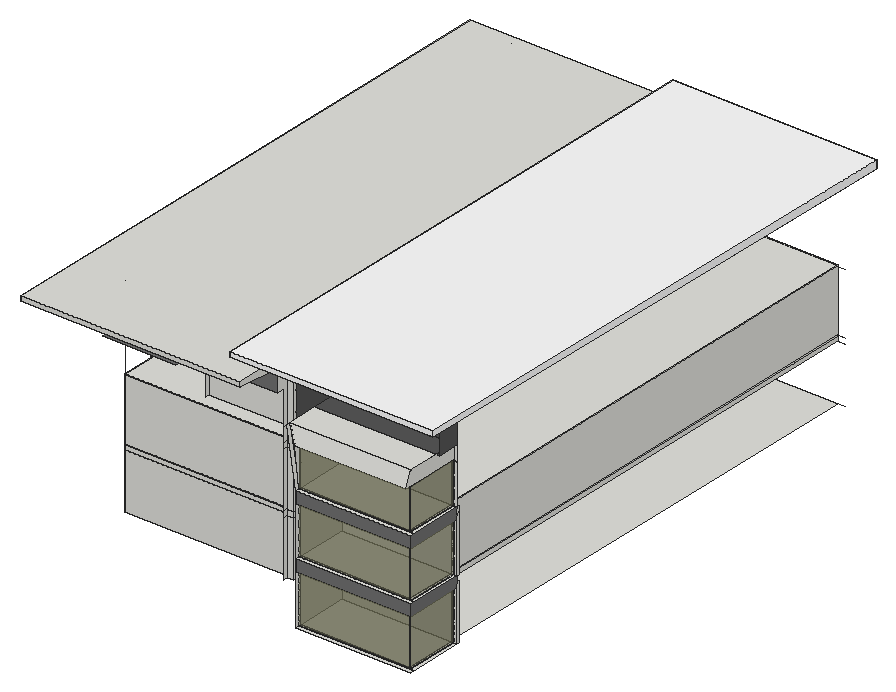
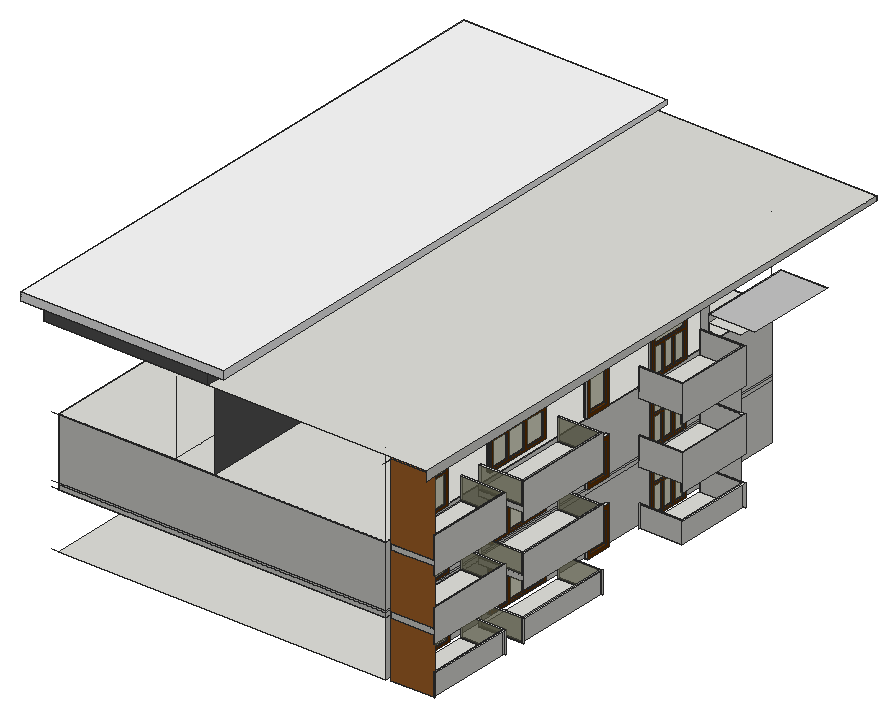
# SketchUp Ruby script. Lengths in inches.
U = 1.inch
M = Sketchup.active_model
def pt(a) = Geom::Point3d.new(a.map { |v| v * U })
def face(e, loops, mat)
  f = e.add_face(loops[0].map { |a| pt(a) })
  loops[1..].each { |l| e.add_face(l.map { |a| pt(a) }).erase! }
  f.material = f.back_material = mat if mat
  f
end
# faces: each face lists its corners as indices into pts; further lists are holes
def faces(e, pts, list, mat = nil) = list.each { |f| face(e, (f[0].is_a?(Array) ? f : [f]).map { |l| l.map { |i| pts[i] } }, mat) }
# xy, xz, yz: faces in a plane at the given z, y or x. An outline is a flat list of corners, or four numbers for a rectangle; further outlines are holes
def ring(l) = l.size == 4 ? [[l[0], l[1]], [l[2], l[1]], [l[2], l[3]], [l[0], l[3]]] : l.each_slice(2).to_a
def flat(e, list, mat, &to3) = list.each { |f| face(e, (f[0].is_a?(Array) ? f : [f]).map { |l| ring(l).map { |u, v| to3.(u, v) } }, mat) }
def xy(e, z, list, mat = nil) = flat(e, list, mat) { |x, y| [x, y, z] }
def xz(e, y, list, mat = nil) = flat(e, list, mat) { |x, z| [x, y, z] }
def yz(e, x, list, mat = nil) = flat(e, list, mat) { |y, z| [x, y, z] }
def lines(e, pts, list) = list.each { |a, b| e.add_line(pt(pts[a]), pt(pts[b])) }
# prism: a flat outline (further loops are holes) pulled along v
def prism(e, loops, v, mat = nil)
  f = face(e, loops, mat); d = Geom::Vector3d.new(v.map { |x| x * U })
  f.pushpull(f.normal.samedirection?(d) ? d.length : -d.length)
end
def box(e, o, s, mat = nil) = prism(e, [[o, [o[0] + s[0], o[1], o[2]], [o[0] + s[0], o[1] + s[1], o[2]], [o[0], o[1] + s[1], o[2]]]], [0, 0, s[2]], mat)
def at(x, y, z, deg = 0) = Geom::Transformation.translation(pt([x, y, z])) * Geom::Transformation.rotation(ORIGIN, Z_AXIS, deg.degrees)
def axes(o, x, y, z) = Geom::Transformation.new([*x, 0, *y, 0, *z, 0, *pt(o).to_a, 1])
def part(name) = M.definitions.add(name)
# library, detail: a bought-in or finely detailed component or shape, given as its bounding box
def library(name, o, s) = part(name).tap { |d| box(d.entities, o, s) }
def detail(e, o, s) = box(e.add_group.entities, o, s)
def put(e, d, t, mat = nil) = e.add_instance(d, t).tap { |i| i.material = mat if mat }
def group(e, t, mat = nil) = e.add_group.tap { |g| g.transformation = t; g.material = mat if mat }.entities
root = M.entities
M.materials.add("[Color A08]").color = [102, 50, 0]
M.materials.add("[Color M00]").color = [255, 255, 255]
M.materials.add("[Color M02]").color = [198, 198, 198]
M.materials.add("[Color M05]").color = [114, 114, 114]
M.materials.add("[Color M06]").color = [86, 86, 86]
M.materials.add("[Translucent Glass Gray]").color = [128, 128, 99]
M.materials["[Translucent Glass Gray]"].alpha = 0.5
M.materials.add("[Translucent Glass Gray]1").color = [128, 128, 95]
M.materials["[Translucent Glass Gray]1"].alpha = 0.5
M.materials.add("[Wood Bamboo]").color = [177, 105, 43]
c1 = part("Group\#2")
xy(c1.entities,0,[[0,0,3.1875,51.25]],"[Color A08]")
xy(c1.entities,5.52,[[0,5.52,3.1875,45.73]],"[Color A08]")
xy(c1.entities,59.16,[[0,5.52,3.1875,45.73]],"[Color A08]")
xy(c1.entities,64.6875,[[0,0,3.1875,51.25]],"[Color A08]")
xz(c1.entities,0,[[0,0,3.1875,64.6875]],"[Color A08]")
xz(c1.entities,5.52,[[0,5.52,3.1875,59.16]],"[Color A08]")
xz(c1.entities,45.73,[[0,5.52,3.1875,59.16]],"[Color A08]")
xz(c1.entities,51.25,[[0,0,3.1875,64.6875]],"[Color A08]")
yz(c1.entities,0,[[[0,0,51.25,64.6875],[5.52,5.52,45.73,59.16]]],"[Color A08]")
yz(c1.entities,3.1875,[[[0,0,51.25,64.6875],[5.52,5.52,45.73,59.16]]],"[Color A08]")
yz(c1.entities,3.1875,[[5.52,5.52,45.73,59.16]],"[Translucent Glass Gray]1")
c2 = part("Group\#1")
xy(c2.entities,0,[[0,0,10.1875,224.125]],"[Color A08]")
xy(c2.entities,8.5,[[0,8.5,10.1875,78.41],[0,83.11,10.1875,147.98],[0,152.67,10.1875,215.625]],"[Color A08]")
xy(c2.entities,168.57,[[0,8.5,10.1875,78.41],[0,83.11,10.1875,147.98],[0,152.67,10.1875,215.625]],"[Color A08]")
xy(c2.entities,174.05,[[0,8.5,10.1875,215.625]],"[Color A08]")
xy(c2.entities,240.6875,[[0,8.5,10.1875,215.625]],"[Color A08]")
xy(c2.entities,249.1875,[[0,0,10.1875,224.125]],"[Color A08]")
xz(c2.entities,0,[[0,0,10.1875,249.1875]],"[Color A08]")
xz(c2.entities,8.5,[[0,8.5,10.1875,168.57],[0,174.05,10.1875,240.6875]],"[Color A08]")
xz(c2.entities,78.41,[[0,8.5,10.1875,168.57]],"[Color A08]")
xz(c2.entities,83.11,[[0,8.5,10.1875,168.57]],"[Color A08]")
xz(c2.entities,147.98,[[0,8.5,10.1875,168.57]],"[Color A08]")
xz(c2.entities,152.67,[[0,8.5,10.1875,168.57]],"[Color A08]")
xz(c2.entities,215.625,[[0,8.5,10.1875,168.57],[0,174.05,10.1875,240.6875]],"[Color A08]")
xz(c2.entities,224.125,[[0,0,10.1875,249.1875]],"[Color A08]")
yz(c2.entities,0,[[[0,0,224.125,249.1875],[8.5,174.05,215.625,240.6875],[8.5,8.5,78.41,168.57],[83.11,8.5,147.98,168.57],[152.67,8.5,215.625,168.57]]],"[Color A08]")
yz(c2.entities,10.1875,[[[0,0,224.125,249.1875],[8.5,174.05,215.625,240.6875],[8.5,8.5,78.41,168.57],[83.11,8.5,147.98,168.57],[152.67,8.5,215.625,168.57]]],"[Color A08]")
yz(c2.entities,10.1875,[[8.5,8.5,78.41,168.57],[83.11,8.5,147.98,168.57],[152.67,8.5,215.625,168.57],[8.5,174.05,215.625,240.6875]],"[Translucent Glass Gray]1")
xy(root,324,[[686.75,124.9375,933.8125,133.1875],[686.75,133.1875,686.75,137.1875,922.0625,137.1875,922.0625,249.0625,926.0625,249.0625,926.0625,133.1875],[926.0625,133.1875,933.8125,249.0625],[686.75,137.1875,922.0625,249.0625],[215.0625,255.0625,917.0625,1292.9375],
  [115.6,459.83,206.0625,619.9],[115.0625,838.07,206.0625,842.07],[115.0625,842.07,206.0625,1048.01],[115.0625,1048.01,206.0625,1052.01],[115.0625,1098.84,206.0625,1102.84],
  [115.0625,1102.84,206.0625,1289.125]])
xy(root,325.72,[[206.0625,703.45,215.0625,760.27]])
xy(root,328.22,[[206.0625,495.59,215.0625,585.34]])
xy(root,329.92,[[206.0625,1132.12,215.0625,1253.37]])
xy(root,332.84,[[206.0625,872.21,215.0625,1021.83]])
xy(root,372,[[111.0625,455.21,206.0625,455.21,206.0625,459.83,115.6,459.83,115.6,619.9,206.0625,619.9,206.0625,624.125,111.0625,624.125],[111.0625,838.07,115.0625,1052.01],[115.0625,838.07,206.0625,842.07],[115.0625,1048.01,206.0625,1052.01],[111.0625,1098.84,115.0625,1289.125],
  [115.0625,1098.84,206.0625,1102.84]])
xy(root,408.34,[[206.0625,703.45,215.0625,760.27]])
xy(root,417.97,[[206.0625,495.59,215.0625,585.34]])
xy(root,419.28,[[206.0625,872.21,215.0625,1021.83]])
xy(root,426.05,[[206.0625,1132.12,215.0625,1253.37]])
xy(root,427.25,[[111.0625,455.21,115.0625,624.125],[111.0625,838.07,115.0625,1052.01],[111.0625,1098.84,115.0625,1289.125]])
xy(root,431.9375,[[686.75,124.9375,933.8125,133.1875],[926.0625,133.1875,933.8125,249.0625]],"[Color M05]")
xy(root,444,[[686.75,137.1875,922.0625,249.0625],[215.0625,255.0625,917.0625,1292.9375]])
xy(root,444,[[115.0625,455.21,206.0625,624.125],[115.0625,838.07,206.0625,1052.01],[115.0625,1098.84,206.0625,1289.125]],"[Wood Bamboo]")
xy(root,452.375,[[215.0625,255.0625,917.0625,1292.9375]])
xy(root,456,[[686.75,124.9375,933.8125,133.1875],[686.75,133.1875,686.75,137.1875,922.0625,137.1875,922.0625,249.0625,926.0625,249.0625,926.0625,133.1875],[926.0625,133.1875,933.8125,249.0625],[686.75,137.1875,922.0625,249.0625],[114.03,458.47,206.0625,620.39],
  [115.0625,838.07,206.0625,842.07],[115.0625,842.07,206.0625,1048.01],[115.0625,1048.01,206.0625,1052.01],[115.0625,1098.84,206.0625,1102.84],[115.0625,1102.84,206.0625,1289.125]])
xy(root,458.84,[[206.0625,703.45,215.0625,760.27]])
xy(root,461.48,[[206.0625,495.54,215.0625,585.29]])
xy(root,462.44,[[206.0625,1132.73,215.0625,1253.98]])
xy(root,468.03,[[206.0625,872.21,215.0625,1021.83]])
xy(root,497.6875,[[111.0625,838.07,115.0625,1052.01],[115.0625,838.07,206.0625,842.07],[115.0625,1048.01,206.0625,1052.01],[111.0625,1098.84,115.0625,1289.125],[115.0625,1098.84,206.0625,1102.84]])
xy(root,504,[[111.0625,455.21,206.0625,455.21,206.0625,458.47,114.03,458.47,114.03,620.39,206.0625,620.39,206.0625,624.125,111.0625,624.125]])
xy(root,541.47,[[206.0625,703.45,215.0625,760.27]])
xy(root,551.23,[[206.0625,495.54,215.0625,585.29]])
xy(root,554.47,[[206.0625,872.21,215.0625,1021.83]])
xy(root,558.57,[[206.0625,1132.73,215.0625,1253.98]])
xy(root,558.875,[[111.0625,455.21,115.0625,624.125],[111.0625,838.07,115.0625,1052.01],[111.0625,1098.84,115.0625,1289.125]])
xy(root,562.9375,[[686.75,124.9375,933.8125,133.1875],[926.0625,133.1875,933.8125,249.0625]],"[Color M05]")
xy(root,576,[[686.75,137.1875,922.0625,249.0625]])
xy(root,576,[[115.0625,455.21,206.0625,624.125],[115.0625,838.07,206.0625,1052.01],[115.0625,1098.84,206.0625,1289.125]],"[Wood Bamboo]")
xy(root,588,[[686.75,124.9375,933.8125,133.1875],[686.75,133.1875,686.75,137.1875,922.0625,137.1875,922.0625,249.0625,926.0625,249.0625,926.0625,133.1875],[926.0625,133.1875,933.8125,249.0625],[686.75,137.1875,922.0625,249.0625],[114.77,459.9,206.0625,619.85],
  [115.0625,838.07,206.0625,842.07],[115.0625,842.07,206.0625,1048.01],[115.0625,1048.01,206.0625,1052.01],[115.0625,1098.84,206.0625,1102.84],[115.0625,1102.84,206.0625,1289.125]])
xy(root,590.375,[[215.0625,255.0625,582.625,1292.9375],[582.625,255.0625,665.97,1292.9375],[665.97,255.0625,917.0625,1292.9375]])
xy(root,593.81,[[206.0625,1136.9,215.0625,1258.15]])
xy(root,594.11,[[206.0625,494.02,215.0625,583.77]])
xy(root,596.28,[[206.0625,703.45,215.0625,760.27]])
xy(root,607.03,[[206.0625,872.21,215.0625,1021.83]])
xy(root,636,[[121.48,455.1875,189.6875,455.21],[111.0625,455.21,206.0625,455.21,206.0625,459.9,114.77,459.9,114.77,619.85,206.0625,619.85,206.0625,624.125,111.0625,624.125],[111.0625,838.07,115.0625,1052.01],[115.0625,838.07,206.0625,842.07],[115.0625,1048.01,206.0625,1052.01],
  [111.0625,1098.84,115.0625,1289.125],[115.0625,1098.84,206.0625,1102.84]])
xy(root,653.32,[[121.48,295.8125,189.6875,422.4375],[121.48,422.4375,189.6875,454.6875]])
xy(root,653.32,[[121.48,280.0625,189.6875,295.8125]],"[Color M02]")
xy(root,669.38,[[90.2,260.8,189.6875,455.1875]],"[Color M02]")
xy(root,675.82,[[686.75,133.1875,926.0625,133.1875,926.0625,249.0625,922.0625,249.0625,922.0625,137.1875,686.75,137.1875],[686.75,137.1875,922.0625,249.0625]])
xy(root,675.82,[[686.75,121.6,926.0625,133.1875]],"[Color M05]")
xy(root,678.91,[[206.0625,703.45,215.0625,760.27]])
xy(root,683.86,[[206.0625,494.02,215.0625,583.77]])
xy(root,689.93,[[206.0625,1136.9,215.0625,1258.15]])
xy(root,691.09,[[216.14,192.6875,374.07,226.5],[400.94,223.8125,568.625,240.375]],"[Color M05]")
xy(root,693.47,[[206.0625,872.21,215.0625,1021.83]])
xy(root,708,[[665.97,133.1875,926.0625,202.6875]])
xy(root,708,[[665.97,202.6875,926.0625,249.0625],[926.0625,202.6875,933.8125,249.0625]],"[Color M06]")
xy(root,750.75,[[400.94,192.6875,400.94,223.8125,568.625,223.8125,568.625,202.6875]],"[Color M00]")
xy(root,750.75,[[189.6875,192.6875,400.94,249.0625],[400.94,223.8125,568.625,249.0625],[189.6875,249.0625,206.0625,455.21]],"[Color M05]")
xy(root,750.75,[[568.625,202.6875,582.625,249.0625]],"[Color M06]")
xy(root,750.75,[[189.6875,455.21,206.0625,1289.125,206.0625,455.21]],"[Wood Bamboo]")
xy(root,771,[[111.0625,103.4375,582.625,103.4375,582.625,249.0625,933.8125,249.0625,933.8125,1311.875,111.0625,1311.875]])
xy(root,792.25,[[933.8125,202.6875,933.8125,1311.875,985.25,1311.875]],"[Color M00]")
xy(root,792.25,[[582.625,202.6875,933.8125,1311.875]],"[Color M06]")
xy(root,809.5625,[[548.25,119.625,985.25,1311.875]],"[Color M00]")
xz(root,103.4375,[[111.0625,760.875,582.625,771]])
xz(root,119.625,[[548.25,798.83,985.25,809.5625]],"[Color M00]")
xz(root,124.9375,[[686.75,431.9375,933.8125,456],[686.75,562.9375,933.8125,588]],"[Color M05]")
xz(root,133.1875,[[686.75,324,926.0625,431.9375],[686.75,456,926.0625,562.9375],[686.75,588,926.0625,675.82]],"[Translucent Glass Gray]")
xz(root,137.1875,[[686.75,431.9375,922.0625,444],[686.75,562.9375,922.0625,576]])
xz(root,137.1875,[[686.75,324,922.0625,431.9375],[686.75,456,922.0625,562.9375],[686.75,588,922.0625,675.82]],"[Translucent Glass Gray]")
xz(root,223.8125,[[400.94,691.09,568.625,750.75]],"[Color M05]")
xz(root,249.0625,[[568.625,324,582.625,444],[686.75,324,922.0625,444],[922.0625,324,926.0625,431.9375],[926.0625,324,933.8125,431.9375],[922.0625,431.9375,933.8125,444],
  [568.625,444,582.625,456],[568.625,456,582.625,576],[922.0625,456,926.0625,562.9375],[926.0625,456,933.8125,562.9375],[568.625,576,582.625,588],
  [568.625,588,582.625,750.75],[686.75,588,922.0625,675.82],[922.0625,588,926.0625,675.82],[926.0625,588,933.8125,675.82],[400.94,617.75,568.625,750.75],
  [926.0625,675.82,933.8125,708]])
xz(root,249.0625,[[686.75,456,922.0625,576]],"[Color M00]")
xz(root,249.0625,[[665.97,708,933.8125,771]],"[Color M06]")
xz(root,249.0625,[[922.0625,562.9375,933.8125,576]],"[Translucent Glass Gray]")
xz(root,255.0625,[[215.0625,324,582.625,444],[582.625,324,665.97,444],[665.97,324,933.8125,444],[215.0625,444,582.625,452.375],[582.625,444,665.97,452.375],
  [665.97,444,917.0625,452.375],[215.0625,452.375,582.625,456],[582.625,452.375,665.97,456],[665.97,452.375,917.0625,456],[215.0625,456,582.625,588],
  [582.625,456,665.97,588],[917.0625,456,933.8125,588],[215.0625,588,582.625,590.375],[582.625,588,665.97,590.375],[665.97,588,917.0625,590.375]])
xz(root,255.0625,[[665.97,456,917.0625,588]],"[Translucent Glass Gray]")
xz(root,455.21,[[111.0625,324,121.48,372],[121.48,324,189.6875,372],[189.6875,324,206.0625,372],[121.48,372,189.6875,444],[189.6875,372,206.0625,444],
  [111.0625,427.25,115.0625,427.25,115.0625,444,121.48,444,121.48,456,111.0625,456],[121.48,444,189.6875,456],[189.6875,444,206.0625,456],[111.0625,456,121.48,504],[121.48,456,189.6875,504],
  [189.6875,456,206.0625,504],[121.48,504,189.6875,576],[189.6875,504,206.0625,576],[111.0625,558.875,115.0625,558.875,115.0625,576,121.48,576,121.48,588,111.0625,588],[121.48,576,189.6875,588],
  [189.6875,576,206.0625,588],[111.0625,588,121.48,636],[121.48,588,189.6875,636],[189.6875,588,206.0625,636],[189.6875,636,206.0625,750.75]])
xz(root,458.47,[[114.03,456,206.0625,504]])
xz(root,459.83,[[115.6,324,206.0625,372]])
xz(root,459.9,[[114.77,588,206.0625,636]])
xz(root,494.02,[[206.0625,594.11,215.0625,683.86]])
xz(root,495.54,[[206.0625,461.48,215.0625,551.23]])
xz(root,495.59,[[206.0625,328.22,215.0625,417.97]])
xz(root,583.77,[[206.0625,594.11,215.0625,683.86]])
xz(root,585.29,[[206.0625,461.48,215.0625,551.23]])
xz(root,585.34,[[206.0625,328.22,215.0625,417.97]])
xz(root,619.85,[[114.77,588,206.0625,636]])
xz(root,619.9,[[115.6,324,206.0625,372]])
xz(root,620.39,[[114.03,456,206.0625,504]])
xz(root,624.125,[[111.0625,427.25,111.0625,504,206.0625,504,206.0625,444,115.0625,444,115.0625,427.25],[111.0625,558.875,111.0625,636,206.0625,636,206.0625,576,115.0625,576,115.0625,558.875]])
xz(root,703.45,[[206.0625,325.72,215.0625,408.34],[206.0625,458.84,215.0625,541.47],[206.0625,596.28,215.0625,678.91]])
xz(root,760.27,[[206.0625,325.72,215.0625,408.34],[206.0625,458.84,215.0625,541.47],[206.0625,596.28,215.0625,678.91]])
xz(root,838.07,[[111.0625,324,115.0625,372],[111.0625,427.25,115.0625,427.25,115.0625,444,206.0625,444,206.0625,456,111.0625,456],[111.0625,456,115.0625,497.6875],[111.0625,558.875,115.0625,558.875,115.0625,576,206.0625,576,206.0625,588,111.0625,588],[111.0625,588,115.0625,636]])
xz(root,838.07,[[115.0625,324,206.0625,372],[115.0625,456,206.0625,497.6875],[115.0625,588,206.0625,636]],"[Translucent Glass Gray]")
xz(root,842.07,[[115.0625,324,206.0625,372],[115.0625,456,206.0625,497.6875],[115.0625,588,206.0625,636]],"[Translucent Glass Gray]")
xz(root,872.21,[[206.0625,332.84,215.0625,419.28],[206.0625,468.03,215.0625,554.47],[206.0625,607.03,215.0625,693.47]])
xz(root,1021.83,[[206.0625,332.84,215.0625,419.28],[206.0625,468.03,215.0625,554.47],[206.0625,607.03,215.0625,693.47]])
xz(root,1048.01,[[115.0625,324,206.0625,372],[115.0625,456,206.0625,497.6875],[115.0625,588,206.0625,636]],"[Translucent Glass Gray]")
xz(root,1052.01,[[111.0625,324,115.0625,372],[111.0625,427.25,111.0625,456,206.0625,456,206.0625,444,115.0625,444,115.0625,427.25],[111.0625,456,115.0625,497.6875],[111.0625,558.875,111.0625,588,206.0625,588,206.0625,576,115.0625,576,115.0625,558.875],[111.0625,588,115.0625,636]])
xz(root,1052.01,[[115.0625,324,206.0625,372],[115.0625,456,206.0625,497.6875],[115.0625,588,206.0625,636]],"[Translucent Glass Gray]")
xz(root,1098.84,[[111.0625,324,115.0625,372],[111.0625,427.25,115.0625,427.25,115.0625,444,206.0625,444,206.0625,456,111.0625,456],[111.0625,456,115.0625,497.6875],[111.0625,558.875,115.0625,558.875,115.0625,576,206.0625,576,206.0625,588,111.0625,588],[111.0625,588,115.0625,636]])
xz(root,1098.84,[[115.0625,324,206.0625,372],[115.0625,456,206.0625,497.6875],[115.0625,588,206.0625,636]],"[Translucent Glass Gray]")
xz(root,1102.84,[[115.0625,324,206.0625,372],[115.0625,456,206.0625,497.6875],[115.0625,588,206.0625,636]],"[Translucent Glass Gray]")
xz(root,1132.12,[[206.0625,329.92,215.0625,426.05]])
xz(root,1132.73,[[206.0625,462.44,215.0625,558.57]])
xz(root,1136.9,[[206.0625,593.81,215.0625,689.93]])
xz(root,1253.37,[[206.0625,329.92,215.0625,426.05]])
xz(root,1253.98,[[206.0625,462.44,215.0625,558.57]])
xz(root,1258.15,[[206.0625,593.81,215.0625,689.93]])
xz(root,1289.125,[[111.0625,324,115.0625,372],[111.0625,427.25,111.0625,456,206.0625,456,206.0625,444,115.0625,444,115.0625,427.25],[111.0625,456,115.0625,497.6875],[111.0625,558.875,111.0625,588,206.0625,588,206.0625,576,115.0625,576,115.0625,558.875],[111.0625,588,115.0625,636]])
xz(root,1289.125,[[115.0625,324,206.0625,324,206.0625,444,115.0625,444,115.0625,427.25,111.0625,427.25,111.0625,372,115.0625,372],[115.0625,456,206.0625,456,206.0625,576,115.0625,576,115.0625,558.875,111.0625,558.875,111.0625,497.6875,115.0625,497.6875],[115.0625,588,206.0625,588,206.0625,750.75,111.0625,750.75,111.0625,636,115.0625,636]],"[Wood Bamboo]")
xz(root,1292.9375,[[215.0625,444,917.0625,452.375],[215.0625,452.375,917.0625,456],[215.0625,456,917.0625,588],[215.0625,588,917.0625,590.375]])
xz(root,1311.875,[[548.25,792.25,985.25,809.5625]],"[Color M00]")
xz(root,1311.875,[[582.625,771,933.8125,792.25]],"[Color M06]")
yz(root,111.0625,[[455.21,427.25,624.125,504],[838.07,427.25,1052.01,497.6875],[1098.84,427.25,1289.125,497.6875],[455.21,558.875,624.125,636],[838.07,558.875,1052.01,636],
  [1098.84,558.875,1289.125,636],[1289.125,750.75,103.4375,760.875,103.4375,771,1311.875,771,1311.875,750.75]])
yz(root,114.03,[[458.47,456,620.39,504]])
yz(root,114.77,[[459.9,588,619.85,636]])
yz(root,115.0625,[[838.07,324,842.07,372],[842.07,324,1048.01,372],[1048.01,324,1052.01,372],[1098.84,324,1102.84,372],[1102.84,324,1289.125,372],
  [455.21,427.25,624.125,444],[838.07,427.25,1052.01,444],[1098.84,427.25,1289.125,444],[838.07,456,842.07,497.6875],[842.07,456,1048.01,497.6875],
  [1048.01,456,1052.01,497.6875],[1098.84,456,1102.84,497.6875],[1102.84,456,1289.125,497.6875],[455.21,558.875,624.125,576],[838.07,558.875,1052.01,576],
  [1098.84,558.875,1289.125,576],[838.07,588,842.07,636],[842.07,588,1048.01,636],[1048.01,588,1052.01,636],[1098.84,588,1102.84,636],
  [1102.84,588,1289.125,636]])
yz(root,115.6,[[459.83,324,619.9,372]])
yz(root,189.6875,[[455.1875,636,455.21,653.32],[280.0625,653.32,422.4375,653.32,418.84,669.38,260.8,669.38],[422.4375,653.32,418.84,669.38,454.63,669.38,454.6875,653.32],[454.6875,653.32,454.63,669.38,455.05,669.38,455.0625,653.32],[455.0625,653.32,455.05,669.38,455.1875,669.38,455.1875,653.32]])
yz(root,206.0625,[[455.21,324,459.83,372],[619.9,324,624.125,372],[838.07,324,842.07,372],[1048.01,324,1052.01,372],[1098.84,324,1102.84,372],
  [1098.84,444,1289.125,456],[455.21,456,458.47,504],[620.39,456,624.125,504],[838.07,456,842.07,497.6875],[1048.01,456,1052.01,497.6875],
  [1098.84,456,1102.84,497.6875],[1098.84,576,1289.125,588],[455.21,588,459.9,636],[619.85,588,624.125,636],[838.07,588,842.07,636],
  [1048.01,588,1052.01,636],[1098.84,588,1102.84,636]])
yz(root,215.0625,[[[255.0625,324,1292.9375,444],[872.21,332.84,1021.83,419.28],[1132.12,329.92,1253.37,426.05],[495.59,328.22,585.34,417.97],[703.45,325.72,760.27,408.34]],[255.0625,444,1292.9375,452.375],[255.0625,452.375,1292.9375,456],[[255.0625,456,1292.9375,588],[872.21,468.03,1021.83,554.47],[1132.73,462.44,1253.98,558.57],[495.54,461.48,585.29,551.23],[703.45,458.84,760.27,541.47]],[255.0625,588,1292.9375,590.375]])
yz(root,400.94,[[240.375,617.75,249.0625,617.75,249.0625,750.75,223.8125,750.75,223.8125,691.09,240.375,691.09]])
yz(root,548.25,[[1311.875,792.25,119.625,798.83,119.625,809.5625,1311.875,809.5625]],"[Color M00]")
yz(root,568.625,[[240.375,324,249.0625,444],[240.375,444,249.0625,456],[240.375,456,249.0625,576],[240.375,576,249.0625,588],[240.375,588,249.0625,617.75],
  [240.375,617.75,240.375,691.09,223.8125,691.09,223.8125,750.75,249.0625,750.75,249.0625,617.75]])
yz(root,582.625,[[249.0625,324,255.0625,444],[249.0625,444,255.0625,456],[249.0625,456,255.0625,576],[249.0625,576,255.0625,588],[249.0625,588,255.0625,771],
  [202.6875,750.75,202.6875,771,103.4375,771,103.4375,760.875]])
yz(root,582.625,[[255.0625,590.375,255.0625,771,202.6875,771,202.6875,792.25,1311.875,792.25,1311.875,771,1292.9375,771,1292.9375,590.375],[202.6875,750.75,249.0625,771]],"[Color M06]")
yz(root,686.75,[[125.3125,324,133.1875,431.9375],[133.1875,324,137.1875,431.9375],[137.1875,324,249.0625,444],[124.9375,431.9375,125.3125,456],[125.3125,456,133.1875,562.9375],
  [133.1875,456,137.1875,562.9375],[137.1875,456,249.0625,576],[124.9375,562.9375,125.3125,588],[133.1875,588,133.1875,675.82,121.6,675.82],[133.1875,588,137.1875,675.82],
  [137.1875,588,249.0625,675.82]])
yz(root,917.0625,[[255.0625,444,1292.9375,452.375],[255.0625,452.375,1292.9375,456],[255.0625,456,1292.9375,588],[255.0625,588,1292.9375,590.375]])
yz(root,922.0625,[[137.1875,431.9375,249.0625,444],[137.1875,562.9375,249.0625,576]])
yz(root,922.0625,[[137.1875,324,249.0625,431.9375],[137.1875,456,249.0625,562.9375],[137.1875,588,249.0625,675.82]],"[Translucent Glass Gray]")
yz(root,926.0625,[[121.6,675.82,249.0625,675.82,249.0625,708,133.1875,708]])
yz(root,926.0625,[[133.1875,324,249.0625,431.9375],[133.1875,456,249.0625,562.9375],[133.1875,588,249.0625,675.82]],"[Translucent Glass Gray]")
yz(root,933.8125,[[249.0625,324,255.0625,444],[249.0625,456,255.0625,576],[249.0625,576,255.0625,588]])
yz(root,933.8125,[[124.9375,431.9375,249.0625,456],[124.9375,562.9375,249.0625,588]],"[Color M05]")
yz(root,933.8125,[[202.6875,708,249.0625,708,249.0625,771,1311.875,771,1311.875,792.25,202.6875,792.25]],"[Color M06]")
yz(root,985.25,[[1311.875,792.25,1311.875,809.5625,119.625,809.5625,119.625,798.83]],"[Color M00]")
p = [[686.75,121.6,675.82],[665.97,133.1875,708],[686.75,133.1875,588],[665.97,125.3125,708],[686.75,125.3125,588],[189.6875,280.0625,653.32],
  [189.6875,260.8,669.38],[90.2,260.8,669.38],[121.48,280.0625,653.32],[926.0625,121.6,675.82],[926.0625,133.1875,708],[111.0625,1289.125,750.75],
  [206.0625,1289.125,750.75],[111.0625,103.4375,760.875],[189.6875,455.21,750.75],[189.6875,192.6875,750.75],[400.94,192.6875,750.75],[582.625,103.4375,760.875],
  [189.6875,249.0625,750.75],[568.625,202.6875,750.75],[582.625,202.6875,750.75],[548.25,1311.875,792.25],[582.625,1311.875,792.25],[548.25,119.625,798.83],
  [582.625,202.6875,792.25],[933.8125,202.6875,792.25],[985.25,119.625,798.83],[985.25,1311.875,792.25],[121.48,455.1875,653.32],[121.48,454.6875,653.32],
  [917.0625,1292.9375,456],[933.8125,1292.9375,456],[215.0625,1292.9375,590.375],[215.0625,1292.9375,771],[215.0625,255.0625,590.375],[215.0625,255.0625,771],
  [206.0625,1311.875,750.75],[917.0625,1292.9375,588],[933.8125,1292.9375,588],[917.0625,1292.9375,444],[933.8125,1292.9375,444],[917.0625,1292.9375,324],
  [933.8125,1292.9375,324],[665.97,1292.9375,750.75],[665.97,1292.9375,590.375],[665.97,249.0625,750.75],[665.97,202.6875,750.75]]
faces(root,p,[[0,1,2],[2,1,3,4],[9,10,1,0]])
faces(root,p,[[5,6,7,8]],"[Color M02]")
faces(root,p,[[11,12,13],[14,13,12],[14,18,15,13]],"[Wood Bamboo]")
faces(root,p,[[13,15,16,17],[19,17,16],[20,17,19],[21,22,23],[24,23,22],[23,24,25,26],[27,26,25]],"[Color M00]")
lines(root,p,[[28,29],[30,31],[32,33],[34,35],[12,36],[37,38],[39,40],[41,42],[43,44],[45,46]])
put(root,c1,axes([206.0625,703.45,324.66],[2.19,0,0],[0,1.10854,0],[0,0,1.27]))
put(root,c2,axes([206.0625,495.59,328.22],[0.56448,0,0],[0,0.40045,0],[0,0,0.36017]))
put(root,c2,axes([206.0625,1132.12,329.92],[0.3,0,0],[0,0.54099,0],[0,0,0.38575]))
put(root,c2,axes([206.0625,872.21,332.84],[0.504,0,0],[0,0.6676,0],[0,0,0.34688]))
put(root,c1,axes([206.0625,703.45,458.84],[2.19,0,0],[0,1.10854,0],[0,0,1.27]))
put(root,c2,axes([206.0625,495.54,461.48],[0.56448,0,0],[0,0.40045,0],[0,0,0.36017]))
put(root,c2,axes([206.0625,1132.73,462.44],[0.3,0,0],[0,0.54099,0],[0,0,0.38575]))
put(root,c2,axes([206.0625,872.21,468.03],[0.504,0,0],[0,0.6676,0],[0,0,0.34688]))
put(root,c2,axes([206.0625,1136.9,593.81],[0.3,0,0],[0,0.54099,0],[0,0,0.38575]))
put(root,c2,axes([206.0625,494.02,594.11],[0.56448,0,0],[0,0.40045,0],[0,0,0.36017]))
put(root,c1,axes([206.0625,703.45,596.28],[2.19,0,0],[0,1.10854,0],[0,0,1.27]))
put(root,c2,axes([206.55,872.21,607.03],[0.504,0,0],[0,0.6676,0],[0,0,0.34688]))
